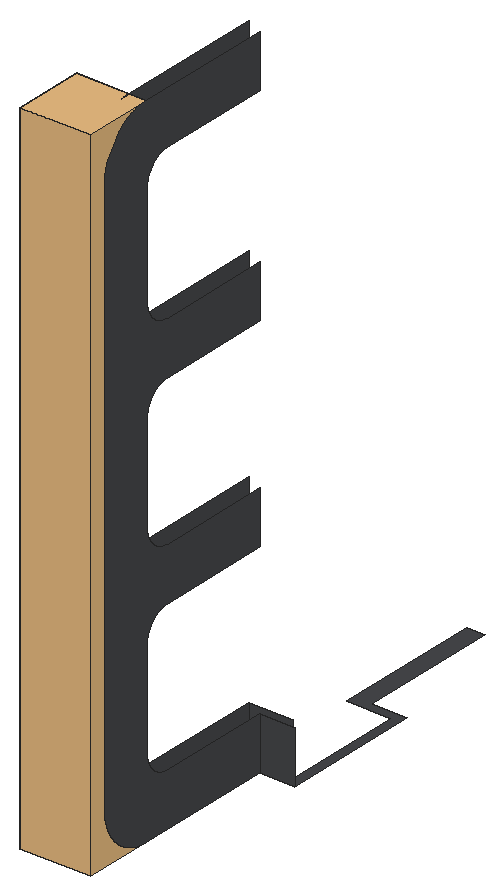
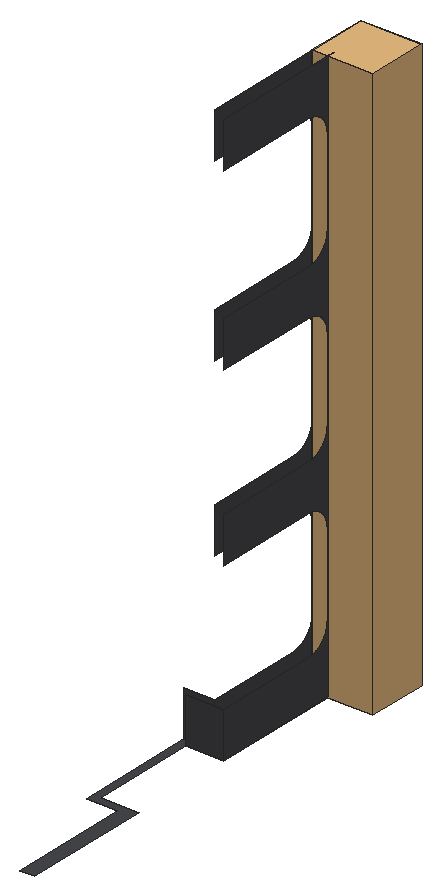
# SketchUp Ruby script. Lengths in inches.
U = 1.inch
M = Sketchup.active_model
def pt(a) = Geom::Point3d.new(a.map { |v| v * U })
def face(e, loops, mat)
  f = e.add_face(loops[0].map { |a| pt(a) })
  loops[1..].each { |l| e.add_face(l.map { |a| pt(a) }).erase! }
  f.material = f.back_material = mat if mat
  f
end
# faces: each face lists its corners as indices into pts; further lists are holes
def faces(e, pts, list, mat = nil) = list.each { |f| face(e, (f[0].is_a?(Array) ? f : [f]).map { |l| l.map { |i| pts[i] } }, mat) }
# xy, xz, yz: faces in a plane at the given z, y or x. An outline is a flat list of corners, or four numbers for a rectangle; further outlines are holes
def ring(l) = l.size == 4 ? [[l[0], l[1]], [l[2], l[1]], [l[2], l[3]], [l[0], l[3]]] : l.each_slice(2).to_a
def flat(e, list, mat, &to3) = list.each { |f| face(e, (f[0].is_a?(Array) ? f : [f]).map { |l| ring(l).map { |u, v| to3.(u, v) } }, mat) }
def xy(e, z, list, mat = nil) = flat(e, list, mat) { |x, y| [x, y, z] }
def xz(e, y, list, mat = nil) = flat(e, list, mat) { |x, z| [x, y, z] }
def yz(e, x, list, mat = nil) = flat(e, list, mat) { |y, z| [x, y, z] }
def lines(e, pts, list) = list.each { |a, b| e.add_line(pt(pts[a]), pt(pts[b])) }
# prism: a flat outline (further loops are holes) pulled along v
def prism(e, loops, v, mat = nil)
  f = face(e, loops, mat); d = Geom::Vector3d.new(v.map { |x| x * U })
  f.pushpull(f.normal.samedirection?(d) ? d.length : -d.length)
end
def box(e, o, s, mat = nil) = prism(e, [[o, [o[0] + s[0], o[1], o[2]], [o[0] + s[0], o[1] + s[1], o[2]], [o[0], o[1] + s[1], o[2]]]], [0, 0, s[2]], mat)
def at(x, y, z, deg = 0) = Geom::Transformation.translation(pt([x, y, z])) * Geom::Transformation.rotation(ORIGIN, Z_AXIS, deg.degrees)
def axes(o, x, y, z) = Geom::Transformation.new([*x, 0, *y, 0, *z, 0, *pt(o).to_a, 1])
def part(name) = M.definitions.add(name)
# library, detail: a bought-in or finely detailed component or shape, given as its bounding box
def library(name, o, s) = part(name).tap { |d| box(d.entities, o, s) }
def detail(e, o, s) = box(e.add_group.entities, o, s)
def put(e, d, t, mat = nil) = e.add_instance(d, t).tap { |i| i.material = mat if mat }
def group(e, t, mat = nil) = e.add_group.tap { |g| g.transformation = t; g.material = mat if mat }.entities
root = M.entities
M.materials.add("1432 AP 8245 TAR ROAD").color = [71, 72, 75]
c1 = library("Group\#18",[0,0,-453],[48,48,453])
xy(root,143.79,[[573,143.09,585,143.37],[573,143.37,573,245.37,603,245.37,603,329.37,573,329.37,573,431.37,585,431.37,585,335.37,609,335.37,609,239.37,585,239.37,585,143.37]],"1432 AP 8245 TAR ROAD")
xy(root,143.8,[[573,142.52,585,142.8]],"1432 AP 8245 TAR ROAD")
xz(root,239.37,[[585,143.79,609,179.79]],"1432 AP 8245 TAR ROAD")
xz(root,245.37,[[573,143.79,603,179.79]],"1432 AP 8245 TAR ROAD")
yz(root,573,[[143.09,143.79,142.8,143.8,142.52,143.8,141.96,143.82,141.67,143.83,141.39,143.85,141.11,143.86,140.55,143.9,140.26,143.93,139.98,143.95,139.14,144.04,138.86,144.08,138.58,144.11,138.02,144.19,137.74,144.24,137.46,144.28,136.9,144.38,136.35,144.48,135.79,144.6,135.52,144.66,135.24,144.72,134.97,144.79,134.69,144.85,134.42,144.92,134.14,144.99,133.87,145.07,133.6,145.14,133.06,145.3,132.78,145.38,132.51,145.47,132.25,145.55,131.71,145.73,131.44,145.83,131.18,145.92,130.64,146.12,130.12,146.32,129.85,146.43,129.59,146.53,129.07,146.75,128.8125,146.87,128.56,146.98,128.04,147.22,127.79,147.34,127.53,147.46,127.03,147.72,126.77,147.85,126.52,147.98,126.28,148.11,126.03,148.25,125.78,148.38,125.53,148.52,125.29,148.66,125.04,148.81,124.8,148.95,123.84,149.55,123.61,149.7,123.13,150.02,122.67,150.34,122.4375,150.5,122.21,150.67,121.98,150.83,121.75,151,121.53,151.17,121.31,151.35,121.08,151.52,120.86,151.7,120.42,152.05,120.21,152.23,119.99,152.42,119.78,152.6,119.5625,152.79,119.35,152.98,118.93,153.36,118.73,153.55,118.52,153.74,118.32,153.94,118.11,154.14,117.71,154.54,117.52,154.74,117.32,154.94,117.13,155.15,116.93,155.36,116.74,155.5625,116.55,155.77,116.37,155.98,116.18,156.2,116,156.41,115.8125,156.63,115.63,156.84,115.45,157.0625,115.27,157.28,115.1,157.5,114.92,157.73,114.75,157.95,114.58,158.18,114.41,158.4,114.25,158.63,114.08,158.86,113.92,159.09,113.75,159.32,113.6,159.56,113.4375,159.79,113.28,160.03,113.125,160.26,112.97,160.5,112.67,160.98,112.53,161.22,112.38,161.47,112.24,161.71,112.1,161.96,111.96,162.2,111.82,162.45,111.6875,162.7,111.55,162.95,111.29,163.45,111.17,163.7,111.04,163.95,110.92,164.21,110.8,164.46,110.44,165.24,110.33,165.49,110.22,165.75,110.11,166.02,110,166.28,109.9,166.54,109.79,166.8,109.69,167.07,109.6,167.33,109.5,167.6,109.4,167.86,109.3125,168.13,109.22,168.4,109.13,168.67,109.05,168.9375,108.96,169.21,108.72,170.02,108.65,170.29,108.57,170.57,108.43,171.11,108.36,171.39,108.3,171.66,108.24,171.9375,108.18,172.22,108.12,172.49,108.0625,172.77,108.01,173.05,107.96,173.32,107.86,173.88,107.8125,174.16,107.77,174.44,107.65,175.28,107.62,175.5625,107.59,175.84,107.53,176.4,107.5,176.6875,107.48,176.97,107.44,177.53,107.42,177.8125,107.41,178.1,107.38,178.94,107.375,179.23,107.37,179.51,107.37,561.07,107.375,561.36,107.38,561.64,107.39,561.92,107.4,562.21,107.42,562.77,107.46,563.33,107.48,563.62,107.5,563.9,107.65,565.3,107.77,566.14,107.8125,566.42,107.86,566.7,108.01,567.54,108.0625,567.82,108.12,568.09,108.24,568.65,108.3,568.92,108.36,569.2,108.5,569.74,108.57,570.02,108.65,570.29,108.72,570.5625,108.8,570.84,108.96,571.38,109.05,571.65,109.13,571.92,109.22,572.19,109.3125,572.45,109.4,572.72,109.5,572.99,109.6,573.25,109.69,573.52,109.79,573.78,109.9,574.04,110,574.31,110.44,575.35,110.56,575.61,110.68,575.86,110.8,576.12,111.04,576.63,111.17,576.88,111.29,577.14,111.55,577.64,111.6875,577.89,111.82,578.14,111.96,578.38,112.1,578.63,112.38,579.12,112.53,579.36,112.67,579.6,112.97,580.08,113.28,580.56,113.4375,580.79,113.6,581.03,113.75,581.26,113.92,581.49,114.08,581.72,114.25,581.95,114.41,582.18,114.58,582.41,114.75,582.63,114.92,582.86,115.1,583.08,115.27,583.3,115.63,583.74,115.8125,583.96,116,584.17,116.18,584.39,116.37,584.6,116.55,584.8125,116.74,585.02,116.93,585.23,117.13,585.4375,117.32,585.64,117.52,585.84,117.71,586.05,118.11,586.45,118.32,586.64,118.52,586.84,118.73,587.03,118.93,587.23,119.35,587.61,119.5625,587.8,119.78,587.98,119.99,588.17,120.21,588.35,120.42,588.53,120.86,588.89,121.08,589.0625,121.31,589.24,121.75,589.58,122.21,589.92,122.4375,590.08,122.67,590.25,123.13,590.57,123.37,590.72,123.61,590.88,123.84,591.04,124.08,591.1875,124.32,591.34,124.56,591.49,124.8,591.63,125.04,591.78,125.29,591.92,125.53,592.0625,125.78,592.2,126.03,592.34,126.28,592.47,126.52,592.61,126.77,592.74,127.03,592.87,127.28,593,127.53,593.12,127.79,593.24,128.04,593.37,128.3,593.49,128.56,593.6,128.8125,593.72,129.07,593.83,129.85,594.16,130.12,594.26,130.38,594.37,130.64,594.47,130.91,594.57,131.18,594.66,131.44,594.76,132.25,595.03,132.51,595.12,132.78,595.2,133.06,595.28,133.87,595.52,134.14,595.59,134.42,595.66,134.69,595.73,134.97,595.8,135.24,595.86,135.52,595.93,135.79,595.99,136.07,596.04,136.35,596.1,136.625,596.15,136.9,596.21,137.18,596.26,137.46,596.3,137.74,596.35,138.86,596.51,140.26,596.66,140.55,596.68,141.39,596.74,141.67,596.75,141.96,596.76,142.8,596.79,245.37,596.79,245.37,560.79,160.9,560.79,160.66,560.78,160.43,560.77,160.19,560.75,159.96,560.74,159.72,560.72,159.49,560.69,159.25,560.67,158.79,560.61,158.55,560.57,157.86,560.45,157.4,560.35,157.17,560.29,156.9375,560.24,156.71,560.18,156.48,560.12,156.26,560.05,156.03,559.98,155.81,559.91,155.58,559.84,154.92,559.6,154.26,559.33,154.05,559.24,153.83,559.14,153.62,559.04,153.41,558.9375,153.2,558.83,152.57,558.5,152.17,558.26,151.96,558.14,151.76,558.02,151.57,557.89,151.37,557.76,151.17,557.625,150.98,557.49,150.41,557.07,150.23,556.93,150.04,556.78,149.5,556.33,149.33,556.17,149.15,556.01,148.81,555.69,148.64,555.52,148.48,555.35,148.3125,555.18,148.15,555.01,147.99,554.84,147.84,554.66,147.68,554.48,147.38,554.12,147.23,553.9375,146.95,553.5625,146.81,553.37,146.67,553.18,146.54,552.99,146.4,552.79,146.27,552.6,146.15,552.4,146.02,552.2,145.9,552,145.78,551.79,145.67,551.59,145.55,551.38,145.33,550.96,145.23,550.75,145.02,550.33,144.93,550.11,144.83,549.9,144.65,549.46,144.57,549.24,144.48,549.02,144.4,548.8,144.33,548.58,144.25,548.35,144.18,548.13,144.11,547.9,144.05,547.68,143.98,547.45,143.92,547.22,143.87,546.99,143.8125,546.76,143.76,546.53,143.72,546.3,143.67,546.07,143.59,545.61,143.56,545.375,143.52,545.14,143.49,544.91,143.47,544.67,143.45,544.4375,143.43,544.2,143.41,543.97,143.39,543.73,143.38,543.5,143.375,543.26,143.37,543.03,143.37,473.56,143.375,473.32,143.38,473.09,143.39,472.85,143.41,472.61,143.45,472.15,143.47,471.91,143.49,471.68,143.52,471.44,143.56,471.21,143.59,470.98,143.63,470.74,143.67,470.51,143.72,470.28,143.76,470.05,143.8125,469.82,143.87,469.59,143.92,469.36,143.98,469.13,144.05,468.91,144.11,468.68,144.18,468.45,144.25,468.23,144.33,468.01,144.4,467.78,144.48,467.5625,144.57,467.34,144.65,467.12,144.74,466.9,144.83,466.6875,144.93,466.47,145.02,466.26,145.125,466.04,145.23,465.83,145.33,465.62,145.55,465.2,145.67,465,145.78,464.79,146.02,464.39,146.15,464.1875,146.27,463.99,146.4,463.79,146.54,463.6,146.67,463.4,147.09,462.83,147.23,462.65,147.38,462.46,147.68,462.1,147.84,461.92,147.99,461.75,148.15,461.57,148.3125,461.4,148.48,461.23,148.64,461.0625,148.81,460.9,148.98,460.74,149.15,460.57,149.33,460.42,149.5,460.26,149.68,460.1,150.04,459.8,150.23,459.66,150.41,459.51,150.98,459.09,151.17,458.96,151.57,458.7,151.76,458.57,151.96,458.44,152.17,458.32,152.37,458.2,152.57,458.09,152.78,457.97,153.2,457.75,153.83,457.45,154.05,457.35,154.26,457.25,154.7,457.07,154.92,456.99,155.14,456.9,155.36,456.82,155.58,456.75,155.81,456.67,156.03,456.6,156.26,456.53,156.48,456.47,156.71,456.41,156.9375,456.35,157.17,456.29,158.09,456.09,158.55,456.01,158.79,455.98,159.25,455.92,159.49,455.89,159.72,455.87,159.96,455.85,160.19,455.83,160.43,455.82,160.66,455.81,160.9,455.8,161.13,455.79,245.37,455.79,245.37,419.79,160.9,419.79,160.66,419.78,160.43,419.77,160.19,419.75,159.96,419.74,159.72,419.72,159.49,419.69,159.25,419.67,158.79,419.61,158.55,419.57,157.86,419.45,157.4,419.35,157.17,419.29,156.9375,419.24,156.71,419.18,156.48,419.12,156.26,419.05,156.03,418.98,155.81,418.91,155.58,418.84,154.92,418.6,154.26,418.33,154.05,418.24,153.83,418.14,153.62,418.04,153.41,417.9375,153.2,417.83,152.57,417.5,152.17,417.26,151.96,417.14,151.76,417.02,151.57,416.89,151.37,416.76,151.17,416.625,150.98,416.49,150.41,416.07,150.23,415.93,150.04,415.78,149.5,415.33,149.33,415.17,149.15,415.01,148.81,414.69,148.64,414.52,148.48,414.35,148.3125,414.18,148.15,414.01,147.99,413.84,147.84,413.66,147.68,413.48,147.38,413.12,147.23,412.9375,146.95,412.5625,146.81,412.37,146.67,412.18,146.54,411.99,146.4,411.79,146.27,411.6,146.15,411.4,146.02,411.2,145.9,411,145.78,410.79,145.67,410.59,145.55,410.38,145.33,409.96,145.23,409.75,145.02,409.33,144.93,409.11,144.83,408.9,144.65,408.46,144.57,408.24,144.48,408.02,144.4,407.8,144.33,407.58,144.25,407.35,144.18,407.13,144.11,406.9,144.05,406.68,143.98,406.45,143.92,406.22,143.87,405.99,143.8125,405.76,143.76,405.53,143.72,405.3,143.67,405.07,143.59,404.61,143.56,404.375,143.52,404.14,143.49,403.91,143.47,403.67,143.45,403.4375,143.43,403.2,143.41,402.97,143.39,402.73,143.38,402.5,143.375,402.26,143.37,402.03,143.37,335.56,143.375,335.32,143.38,335.09,143.39,334.85,143.41,334.61,143.45,334.15,143.47,333.91,143.49,333.68,143.52,333.44,143.56,333.21,143.59,332.98,143.63,332.74,143.67,332.51,143.72,332.28,143.76,332.05,143.8125,331.82,143.87,331.59,143.92,331.36,143.98,331.13,144.05,330.91,144.11,330.68,144.18,330.45,144.25,330.23,144.33,330.01,144.4,329.78,144.48,329.5625,144.57,329.34,144.65,329.12,144.74,328.9,144.83,328.6875,144.93,328.47,145.02,328.26,145.125,328.04,145.23,327.83,145.33,327.62,145.55,327.2,145.67,327,145.78,326.79,146.02,326.39,146.15,326.1875,146.27,325.99,146.4,325.79,146.54,325.6,146.67,325.4,147.09,324.83,147.23,324.65,147.38,324.46,147.68,324.1,147.84,323.92,147.99,323.75,148.15,323.57,148.3125,323.4,148.48,323.23,148.64,323.0625,148.81,322.9,148.98,322.74,149.15,322.57,149.33,322.42,149.5,322.26,149.68,322.1,150.04,321.8,150.23,321.66,150.41,321.51,150.98,321.09,151.17,320.96,151.57,320.7,151.76,320.57,151.96,320.44,152.17,320.32,152.37,320.2,152.57,320.09,152.78,319.97,153.2,319.75,153.83,319.45,154.05,319.35,154.26,319.25,154.7,319.07,154.92,318.99,155.14,318.9,155.36,318.82,155.58,318.75,155.81,318.67,156.03,318.6,156.26,318.53,156.48,318.47,156.71,318.41,156.9375,318.35,157.17,318.29,158.09,318.09,158.55,318.01,158.79,317.98,159.25,317.92,159.49,317.89,159.72,317.87,159.96,317.85,160.19,317.83,160.43,317.82,160.66,317.81,160.9,317.8,161.13,317.79,245.37,317.79,245.37,281.79,160.9,281.79,160.66,281.78,160.43,281.77,160.19,281.75,159.96,281.74,159.72,281.72,159.49,281.69,159.25,281.67,158.79,281.61,158.55,281.57,157.86,281.45,157.4,281.35,157.17,281.29,156.9375,281.24,156.71,281.18,156.48,281.12,156.26,281.05,156.03,280.98,155.81,280.91,155.58,280.84,154.92,280.6,154.26,280.33,154.05,280.24,153.83,280.14,153.62,280.04,153.41,279.9375,153.2,279.83,152.57,279.5,152.17,279.26,151.96,279.14,151.76,279.02,151.57,278.89,151.37,278.76,151.17,278.625,150.98,278.49,150.41,278.07,150.23,277.93,150.04,277.78,149.5,277.33,149.33,277.17,149.15,277.01,148.81,276.69,148.64,276.52,148.48,276.35,148.3125,276.18,148.15,276.01,147.99,275.84,147.84,275.66,147.68,275.48,147.38,275.12,147.23,274.9375,146.95,274.5625,146.81,274.37,146.67,274.18,146.54,273.99,146.4,273.79,146.27,273.6,146.15,273.4,146.02,273.2,145.9,273,145.78,272.79,145.67,272.59,145.55,272.38,145.33,271.96,145.23,271.75,145.02,271.33,144.93,271.11,144.83,270.9,144.65,270.46,144.57,270.24,144.48,270.02,144.4,269.8,144.33,269.58,144.25,269.35,144.18,269.13,144.11,268.9,144.05,268.68,143.98,268.45,143.92,268.22,143.87,267.99,143.8125,267.76,143.76,267.53,143.72,267.3,143.67,267.07,143.59,266.61,143.56,266.375,143.52,266.14,143.49,265.91,143.47,265.67,143.45,265.4375,143.43,265.2,143.41,264.97,143.39,264.73,143.38,264.5,143.375,264.26,143.37,264.03,143.37,197.56,143.375,197.32,143.38,197.09,143.39,196.85,143.41,196.61,143.45,196.15,143.47,195.91,143.49,195.68,143.52,195.44,143.56,195.21,143.59,194.98,143.63,194.74,143.67,194.51,143.72,194.28,143.76,194.05,143.8125,193.82,143.87,193.59,143.92,193.36,143.98,193.13,144.05,192.91,144.11,192.68,144.18,192.45,144.25,192.23,144.33,192.01,144.4,191.78,144.48,191.5625,144.57,191.34,144.65,191.12,144.74,190.9,144.83,190.6875,144.93,190.47,145.02,190.26,145.125,190.04,145.23,189.83,145.33,189.62,145.55,189.2,145.67,189,145.78,188.79,146.02,188.39,146.15,188.1875,146.27,187.99,146.4,187.79,146.54,187.6,146.67,187.4,147.09,186.83,147.23,186.65,147.38,186.46,147.68,186.1,147.84,185.92,147.99,185.75,148.15,185.57,148.3125,185.4,148.48,185.23,148.64,185.0625,148.81,184.9,148.98,184.74,149.15,184.57,149.33,184.42,149.5,184.26,149.68,184.1,150.04,183.8,150.23,183.66,150.41,183.51,150.98,183.09,151.17,182.96,151.57,182.7,151.76,182.57,151.96,182.44,152.17,182.32,152.37,182.2,152.57,182.09,152.78,181.97,153.2,181.75,153.83,181.45,154.05,181.35,154.26,181.25,154.7,181.07,154.92,180.99,155.14,180.9,155.36,180.82,155.58,180.75,155.81,180.67,156.03,180.6,156.26,180.53,156.48,180.47,156.71,180.41,156.9375,180.35,157.17,180.29,158.09,180.09,158.55,180.01,158.79,179.98,159.25,179.92,159.49,179.89,159.72,179.87,159.96,179.85,160.19,179.83,160.43,179.82,160.66,179.81,160.9,179.8,161.13,179.79,245.37,179.79,245.37,143.79]],"1432 AP 8245 TAR ROAD")
yz(root,585,[[143.09,143.79,239.37,143.79,239.37,179.79,161.13,179.79,160.9,179.8,160.66,179.81,160.43,179.82,160.19,179.83,159.96,179.85,159.72,179.87,159.49,179.89,159.25,179.92,158.79,179.98,158.55,180.01,158.09,180.09,157.17,180.29,156.9375,180.35,156.71,180.41,156.48,180.47,156.26,180.53,156.03,180.6,155.81,180.67,155.58,180.75,155.36,180.82,155.14,180.9,154.92,180.99,154.7,181.07,154.26,181.25,154.05,181.35,153.83,181.45,153.2,181.75,152.78,181.97,152.57,182.09,152.37,182.2,152.17,182.32,151.96,182.44,151.76,182.57,151.57,182.7,151.17,182.96,150.98,183.09,150.41,183.51,150.23,183.66,150.04,183.8,149.68,184.1,149.5,184.26,149.33,184.42,149.15,184.57,148.98,184.74,148.81,184.9,148.64,185.0625,148.48,185.23,148.3125,185.4,148.15,185.57,147.99,185.75,147.84,185.92,147.68,186.1,147.38,186.46,147.23,186.65,147.09,186.83,146.67,187.4,146.54,187.6,146.4,187.79,146.27,187.99,146.15,188.1875,146.02,188.39,145.78,188.79,145.67,189,145.55,189.2,145.33,189.62,145.23,189.83,145.125,190.04,145.02,190.26,144.93,190.47,144.83,190.6875,144.74,190.9,144.65,191.12,144.57,191.34,144.48,191.5625,144.4,191.78,144.33,192.01,144.25,192.23,144.18,192.45,144.11,192.68,144.05,192.91,143.98,193.13,143.92,193.36,143.87,193.59,143.8125,193.82,143.76,194.05,143.72,194.28,143.67,194.51,143.63,194.74,143.59,194.98,143.56,195.21,143.52,195.44,143.49,195.68,143.47,195.91,143.45,196.15,143.41,196.61,143.39,196.85,143.38,197.09,143.375,197.32,143.37,197.56,143.37,264.03,143.375,264.26,143.38,264.5,143.39,264.73,143.41,264.97,143.43,265.2,143.45,265.4375,143.47,265.67,143.49,265.91,143.52,266.14,143.56,266.375,143.59,266.61,143.67,267.07,143.72,267.3,143.76,267.53,143.8125,267.76,143.87,267.99,143.92,268.22,143.98,268.45,144.05,268.68,144.11,268.9,144.18,269.13,144.25,269.35,144.33,269.58,144.4,269.8,144.48,270.02,144.57,270.24,144.65,270.46,144.83,270.9,144.93,271.11,145.02,271.33,145.23,271.75,145.33,271.96,145.55,272.38,145.67,272.59,145.78,272.79,145.9,273,146.02,273.2,146.15,273.4,146.27,273.6,146.4,273.79,146.54,273.99,146.67,274.18,146.81,274.37,146.95,274.5625,147.23,274.9375,147.38,275.12,147.68,275.48,147.84,275.66,147.99,275.84,148.15,276.01,148.3125,276.18,148.48,276.35,148.64,276.52,148.81,276.69,149.15,277.01,149.33,277.17,149.5,277.33,150.04,277.78,150.23,277.93,150.41,278.07,150.98,278.49,151.17,278.625,151.37,278.76,151.57,278.89,151.76,279.02,151.96,279.14,152.17,279.26,152.57,279.5,153.2,279.83,153.41,279.9375,153.62,280.04,153.83,280.14,154.05,280.24,154.26,280.33,154.92,280.6,155.58,280.84,155.81,280.91,156.03,280.98,156.26,281.05,156.48,281.12,156.71,281.18,156.9375,281.24,157.17,281.29,157.4,281.35,157.86,281.45,158.55,281.57,158.79,281.61,159.25,281.67,159.49,281.69,159.72,281.72,159.96,281.74,160.19,281.75,160.43,281.77,160.66,281.78,160.9,281.79,239.37,281.79,239.37,317.79,161.13,317.79,160.9,317.8,160.66,317.81,160.43,317.82,160.19,317.83,159.96,317.85,159.72,317.87,159.49,317.89,159.25,317.92,158.79,317.98,158.55,318.01,158.09,318.09,157.17,318.29,156.9375,318.35,156.71,318.41,156.48,318.47,156.26,318.53,156.03,318.6,155.81,318.67,155.58,318.75,155.36,318.82,155.14,318.9,154.92,318.99,154.7,319.07,154.26,319.25,154.05,319.35,153.83,319.45,153.2,319.75,152.78,319.97,152.57,320.09,152.37,320.2,152.17,320.32,151.96,320.44,151.76,320.57,151.57,320.7,151.17,320.96,150.98,321.09,150.41,321.51,150.23,321.66,150.04,321.8,149.68,322.1,149.5,322.26,149.33,322.42,149.15,322.57,148.98,322.74,148.81,322.9,148.64,323.0625,148.48,323.23,148.3125,323.4,148.15,323.57,147.99,323.75,147.84,323.92,147.68,324.1,147.38,324.46,147.23,324.65,147.09,324.83,146.67,325.4,146.54,325.6,146.4,325.79,146.27,325.99,146.15,326.1875,146.02,326.39,145.78,326.79,145.67,327,145.55,327.2,145.33,327.62,145.23,327.83,145.125,328.04,145.02,328.26,144.93,328.47,144.83,328.6875,144.74,328.9,144.65,329.12,144.57,329.34,144.48,329.5625,144.4,329.78,144.33,330.01,144.25,330.23,144.18,330.45,144.11,330.68,144.05,330.91,143.98,331.13,143.92,331.36,143.87,331.59,143.8125,331.82,143.76,332.05,143.72,332.28,143.67,332.51,143.63,332.74,143.59,332.98,143.56,333.21,143.52,333.44,143.49,333.68,143.47,333.91,143.45,334.15,143.41,334.61,143.39,334.85,143.38,335.09,143.375,335.32,143.37,335.56,143.37,402.03,143.375,402.26,143.38,402.5,143.39,402.73,143.41,402.97,143.43,403.2,143.45,403.4375,143.47,403.67,143.49,403.91,143.52,404.14,143.56,404.375,143.59,404.61,143.67,405.07,143.72,405.3,143.76,405.53,143.8125,405.76,143.87,405.99,143.92,406.22,143.98,406.45,144.05,406.68,144.11,406.9,144.18,407.13,144.25,407.35,144.33,407.58,144.4,407.8,144.48,408.02,144.57,408.24,144.65,408.46,144.83,408.9,144.93,409.11,145.02,409.33,145.23,409.75,145.33,409.96,145.55,410.38,145.67,410.59,145.78,410.79,145.9,411,146.02,411.2,146.15,411.4,146.27,411.6,146.4,411.79,146.54,411.99,146.67,412.18,146.81,412.37,146.95,412.5625,147.23,412.9375,147.38,413.12,147.68,413.48,147.84,413.66,147.99,413.84,148.15,414.01,148.3125,414.18,148.48,414.35,148.64,414.52,148.81,414.69,149.15,415.01,149.33,415.17,149.5,415.33,150.04,415.78,150.23,415.93,150.41,416.07,150.98,416.49,151.17,416.625,151.37,416.76,151.57,416.89,151.76,417.02,151.96,417.14,152.17,417.26,152.57,417.5,153.2,417.83,153.41,417.9375,153.62,418.04,153.83,418.14,154.05,418.24,154.26,418.33,154.92,418.6,155.58,418.84,155.81,418.91,156.03,418.98,156.26,419.05,156.48,419.12,156.71,419.18,156.9375,419.24,157.17,419.29,157.4,419.35,157.86,419.45,158.55,419.57,158.79,419.61,159.25,419.67,159.49,419.69,159.72,419.72,159.96,419.74,160.19,419.75,160.43,419.77,160.66,419.78,160.9,419.79,239.37,419.79,239.37,455.79,161.13,455.79,160.9,455.8,160.66,455.81,160.43,455.82,160.19,455.83,159.96,455.85,159.72,455.87,159.49,455.89,159.25,455.92,158.79,455.98,158.55,456.01,158.09,456.09,157.17,456.29,156.9375,456.35,156.71,456.41,156.48,456.47,156.26,456.53,156.03,456.6,155.81,456.67,155.58,456.75,155.36,456.82,155.14,456.9,154.92,456.99,154.7,457.07,154.26,457.25,154.05,457.35,153.83,457.45,153.2,457.75,152.78,457.97,152.57,458.09,152.37,458.2,152.17,458.32,151.96,458.44,151.76,458.57,151.57,458.7,151.17,458.96,150.98,459.09,150.41,459.51,150.23,459.66,150.04,459.8,149.68,460.1,149.5,460.26,149.33,460.42,149.15,460.57,148.98,460.74,148.81,460.9,148.64,461.0625,148.48,461.23,148.3125,461.4,148.15,461.57,147.99,461.75,147.84,461.92,147.68,462.1,147.38,462.46,147.23,462.65,147.09,462.83,146.67,463.4,146.54,463.6,146.4,463.79,146.27,463.99,146.15,464.1875,146.02,464.39,145.78,464.79,145.67,465,145.55,465.2,145.33,465.62,145.23,465.83,145.125,466.04,145.02,466.26,144.93,466.47,144.83,466.6875,144.74,466.9,144.65,467.12,144.57,467.34,144.48,467.5625,144.4,467.78,144.33,468.01,144.25,468.23,144.18,468.45,144.11,468.68,144.05,468.91,143.98,469.13,143.92,469.36,143.87,469.59,143.8125,469.82,143.76,470.05,143.72,470.28,143.67,470.51,143.63,470.74,143.59,470.98,143.56,471.21,143.52,471.44,143.49,471.68,143.47,471.91,143.45,472.15,143.41,472.61,143.39,472.85,143.38,473.09,143.375,473.32,143.37,473.56,143.37,543.03,143.375,543.26,143.38,543.5,143.39,543.73,143.41,543.97,143.43,544.2,143.45,544.4375,143.47,544.67,143.49,544.91,143.52,545.14,143.56,545.375,143.59,545.61,143.67,546.07,143.72,546.3,143.76,546.53,143.8125,546.76,143.87,546.99,143.92,547.22,143.98,547.45,144.05,547.68,144.11,547.9,144.18,548.13,144.25,548.35,144.33,548.58,144.4,548.8,144.48,549.02,144.57,549.24,144.65,549.46,144.83,549.9,144.93,550.11,145.02,550.33,145.23,550.75,145.33,550.96,145.55,551.38,145.67,551.59,145.78,551.79,145.9,552,146.02,552.2,146.15,552.4,146.27,552.6,146.4,552.79,146.54,552.99,146.67,553.18,146.81,553.37,146.95,553.5625,147.23,553.9375,147.38,554.12,147.68,554.48,147.84,554.66,147.99,554.84,148.15,555.01,148.3125,555.18,148.48,555.35,148.64,555.52,148.81,555.69,149.15,556.01,149.33,556.17,149.5,556.33,150.04,556.78,150.23,556.93,150.41,557.07,150.98,557.49,151.17,557.625,151.37,557.76,151.57,557.89,151.76,558.02,151.96,558.14,152.17,558.26,152.57,558.5,153.2,558.83,153.41,558.9375,153.62,559.04,153.83,559.14,154.05,559.24,154.26,559.33,154.92,559.6,155.58,559.84,155.81,559.91,156.03,559.98,156.26,560.05,156.48,560.12,156.71,560.18,156.9375,560.24,157.17,560.29,157.4,560.35,157.86,560.45,158.55,560.57,158.79,560.61,159.25,560.67,159.49,560.69,159.72,560.72,159.96,560.74,160.19,560.75,160.43,560.77,160.66,560.78,160.9,560.79,239.37,560.79,239.37,596.79,142.8,596.79,141.96,596.76,141.67,596.75,141.39,596.74,140.55,596.68,140.26,596.66,138.86,596.51,137.74,596.35,137.46,596.3,137.18,596.26,136.9,596.21,136.625,596.15,136.35,596.1,136.07,596.04,135.79,595.99,135.52,595.93,135.24,595.86,134.97,595.8,134.69,595.73,134.42,595.66,134.14,595.59,133.87,595.52,133.06,595.28,132.78,595.2,132.51,595.12,132.25,595.03,131.44,594.76,131.18,594.66,130.91,594.57,130.64,594.47,130.38,594.37,130.12,594.26,129.85,594.16,129.07,593.83,128.8125,593.72,128.56,593.6,128.3,593.49,128.04,593.37,127.79,593.24,127.53,593.12,127.28,593,127.03,592.87,126.77,592.74,126.52,592.61,126.28,592.47,126.03,592.34,125.78,592.2,125.53,592.0625,125.29,591.92,125.04,591.78,124.8,591.63,124.56,591.49,124.32,591.34,124.08,591.1875,123.84,591.04,123.61,590.88,123.37,590.72,123.13,590.57,122.67,590.25,122.4375,590.08,122.21,589.92,121.75,589.58,121.31,589.24,121.08,589.0625,120.86,588.89,120.42,588.53,120.21,588.35,119.99,588.17,119.78,587.98,119.5625,587.8,119.35,587.61,118.93,587.23,118.73,587.03,118.52,586.84,118.32,586.64,118.11,586.45,117.71,586.05,117.52,585.84,117.32,585.64,117.13,585.4375,116.93,585.23,116.74,585.02,116.55,584.8125,116.37,584.6,116.18,584.39,116,584.17,115.8125,583.96,115.63,583.74,115.27,583.3,115.1,583.08,114.92,582.86,114.75,582.63,114.58,582.41,114.41,582.18,114.25,581.95,114.08,581.72,113.92,581.49,113.75,581.26,113.6,581.03,113.4375,580.79,113.28,580.56,112.97,580.08,112.67,579.6,112.53,579.36,112.38,579.12,112.1,578.63,111.96,578.38,111.82,578.14,111.6875,577.89,111.55,577.64,111.29,577.14,111.17,576.88,111.04,576.63,110.8,576.12,110.68,575.86,110.56,575.61,110.44,575.35,110,574.31,109.9,574.04,109.79,573.78,109.69,573.52,109.6,573.25,109.5,572.99,109.4,572.72,109.3125,572.45,109.22,572.19,109.13,571.92,109.05,571.65,108.96,571.38,108.8,570.84,108.72,570.5625,108.65,570.29,108.57,570.02,108.5,569.74,108.36,569.2,108.3,568.92,108.24,568.65,108.12,568.09,108.0625,567.82,108.01,567.54,107.86,566.7,107.8125,566.42,107.77,566.14,107.65,565.3,107.5,563.9,107.48,563.62,107.46,563.33,107.42,562.77,107.4,562.21,107.39,561.92,107.38,561.64,107.375,561.36,107.37,561.07,107.37,179.51,107.375,179.23,107.38,178.94,107.41,178.1,107.42,177.8125,107.44,177.53,107.48,176.97,107.5,176.6875,107.53,176.4,107.59,175.84,107.62,175.5625,107.65,175.28,107.77,174.44,107.8125,174.16,107.86,173.88,107.96,173.32,108.01,173.05,108.0625,172.77,108.12,172.49,108.18,172.22,108.24,171.9375,108.3,171.66,108.36,171.39,108.43,171.11,108.57,170.57,108.65,170.29,108.72,170.02,108.96,169.21,109.05,168.9375,109.13,168.67,109.22,168.4,109.3125,168.13,109.4,167.86,109.5,167.6,109.6,167.33,109.69,167.07,109.79,166.8,109.9,166.54,110,166.28,110.11,166.02,110.22,165.75,110.33,165.49,110.44,165.24,110.8,164.46,110.92,164.21,111.04,163.95,111.17,163.7,111.29,163.45,111.55,162.95,111.6875,162.7,111.82,162.45,111.96,162.2,112.1,161.96,112.24,161.71,112.38,161.47,112.53,161.22,112.67,160.98,112.97,160.5,113.125,160.26,113.28,160.03,113.4375,159.79,113.6,159.56,113.75,159.32,113.92,159.09,114.08,158.86,114.25,158.63,114.41,158.4,114.58,158.18,114.75,157.95,114.92,157.73,115.1,157.5,115.27,157.28,115.45,157.0625,115.63,156.84,115.8125,156.63,116,156.41,116.18,156.2,116.37,155.98,116.55,155.77,116.74,155.5625,116.93,155.36,117.13,155.15,117.32,154.94,117.52,154.74,117.71,154.54,118.11,154.14,118.32,153.94,118.52,153.74,118.73,153.55,118.93,153.36,119.35,152.98,119.5625,152.79,119.78,152.6,119.99,152.42,120.21,152.23,120.42,152.05,120.86,151.7,121.08,151.52,121.31,151.35,121.53,151.17,121.75,151,121.98,150.83,122.21,150.67,122.4375,150.5,122.67,150.34,123.13,150.02,123.61,149.7,123.84,149.55,124.8,148.95,125.04,148.81,125.29,148.66,125.53,148.52,125.78,148.38,126.03,148.25,126.28,148.11,126.52,147.98,126.77,147.85,127.03,147.72,127.53,147.46,127.79,147.34,128.04,147.22,128.56,146.98,128.8125,146.87,129.07,146.75,129.59,146.53,129.85,146.43,130.12,146.32,130.64,146.12,131.18,145.92,131.44,145.83,131.71,145.73,132.25,145.55,132.51,145.47,132.78,145.38,133.06,145.3,133.6,145.14,133.87,145.07,134.14,144.99,134.42,144.92,134.69,144.85,134.97,144.79,135.24,144.72,135.52,144.66,135.79,144.6,136.35,144.48,136.9,144.38,137.46,144.28,137.74,144.24,138.02,144.19,138.58,144.11,138.86,144.08,139.14,144.04,139.98,143.95,140.26,143.93,140.55,143.9,141.11,143.86,141.39,143.85,141.67,143.83,141.96,143.82,142.52,143.8,142.8,143.8]],"1432 AP 8245 TAR ROAD")
p = [[573,141.11,143.86],[573,141.39,143.85],[585,141.39,143.85],[585,141.11,143.86],[573,141.67,143.83],[585,141.67,143.83],
  [573,141.96,143.82],[585,141.96,143.82],[573,142.24,143.81],[585,142.24,143.81],[573,142.52,143.8],[585,142.52,143.8],
  [573,142.8,143.8],[573,143.09,143.79],[585,143.09,143.79],[585,142.8,143.8],[573,140.55,143.9],[573,140.83,143.88],
  [585,140.83,143.88],[585,140.55,143.9]]
faces(root,p,[[0,1,2,3],[1,4,5,2],[4,6,7,5],[6,8,9,7],[8,10,11,9],[12,13,14,15],[16,17,18,19],[17,0,3,18]],"1432 AP 8245 TAR ROAD")
put(root,c1,at(537,95.37,596.79),"1432 AP 8245 TAR ROAD")
